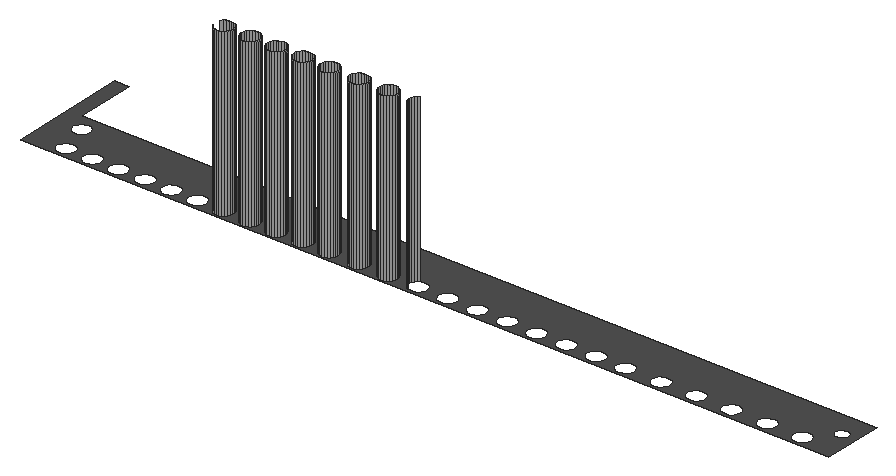
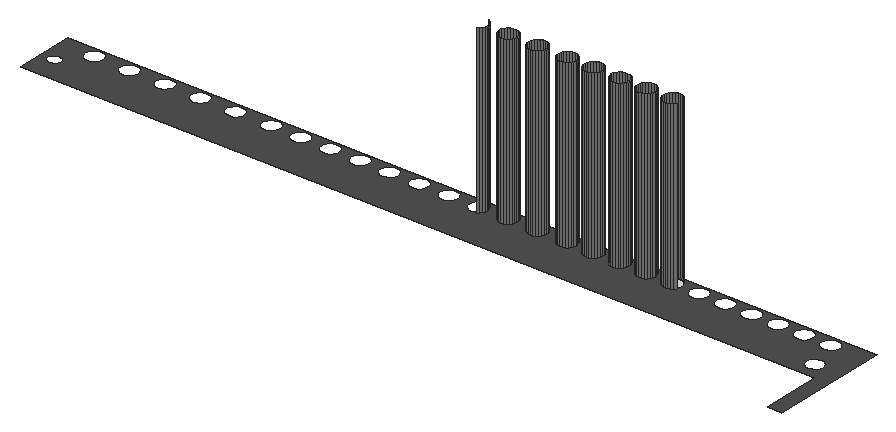
# SketchUp Ruby script. Lengths in inches.
U = 1.inch
M = Sketchup.active_model
def pt(a) = Geom::Point3d.new(a.map { |v| v * U })
def face(e, loops, mat)
  f = e.add_face(loops[0].map { |a| pt(a) })
  loops[1..].each { |l| e.add_face(l.map { |a| pt(a) }).erase! }
  f.material = f.back_material = mat if mat
  f
end
# faces: each face lists its corners as indices into pts; further lists are holes
def faces(e, pts, list, mat = nil) = list.each { |f| face(e, (f[0].is_a?(Array) ? f : [f]).map { |l| l.map { |i| pts[i] } }, mat) }
# xy, xz, yz: faces in a plane at the given z, y or x. An outline is a flat list of corners, or four numbers for a rectangle; further outlines are holes
def ring(l) = l.size == 4 ? [[l[0], l[1]], [l[2], l[1]], [l[2], l[3]], [l[0], l[3]]] : l.each_slice(2).to_a
def flat(e, list, mat, &to3) = list.each { |f| face(e, (f[0].is_a?(Array) ? f : [f]).map { |l| ring(l).map { |u, v| to3.(u, v) } }, mat) }
def xy(e, z, list, mat = nil) = flat(e, list, mat) { |x, y| [x, y, z] }
def xz(e, y, list, mat = nil) = flat(e, list, mat) { |x, z| [x, y, z] }
def yz(e, x, list, mat = nil) = flat(e, list, mat) { |y, z| [x, y, z] }
def lines(e, pts, list) = list.each { |a, b| e.add_line(pt(pts[a]), pt(pts[b])) }
# prism: a flat outline (further loops are holes) pulled along v
def prism(e, loops, v, mat = nil)
  f = face(e, loops, mat); d = Geom::Vector3d.new(v.map { |x| x * U })
  f.pushpull(f.normal.samedirection?(d) ? d.length : -d.length)
end
def box(e, o, s, mat = nil) = prism(e, [[o, [o[0] + s[0], o[1], o[2]], [o[0] + s[0], o[1] + s[1], o[2]], [o[0], o[1] + s[1], o[2]]]], [0, 0, s[2]], mat)
def at(x, y, z, deg = 0) = Geom::Transformation.translation(pt([x, y, z])) * Geom::Transformation.rotation(ORIGIN, Z_AXIS, deg.degrees)
def axes(o, x, y, z) = Geom::Transformation.new([*x, 0, *y, 0, *z, 0, *pt(o).to_a, 1])
def part(name) = M.definitions.add(name)
# library, detail: a bought-in or finely detailed component or shape, given as its bounding box
def library(name, o, s) = part(name).tap { |d| box(d.entities, o, s) }
def detail(e, o, s) = box(e.add_group.entities, o, s)
def put(e, d, t, mat = nil) = e.add_instance(d, t).tap { |i| i.material = mat if mat }
def group(e, t, mat = nil) = e.add_group.tap { |g| g.transformation = t; g.material = mat if mat }.entities
root = M.entities
M.materials.add("[0132_LightGray]").color = [169, 169, 169]
M.materials.add("[0135_DarkGray]").color = [81, 81, 81]
xy(root,638.72,[[270.33,31.93,269.97,31.97,269.64,32.11,269.36,32.33,269.14,32.62,269,32.95,268.95,33.3,269,33.66,269.14,33.99,269.36,34.28,269.64,34.49,269.97,34.63,270.33,34.68,270.68,34.63,271.02,34.49,271.3,34.28,271.52,33.99,271.66,33.66,271.7,33.3,271.66,32.95,271.52,32.62,271.3,32.33,271.02,32.11,270.68,31.97],[274.33,31.93,273.97,31.97,273.64,32.11,273.36,32.33,273.14,32.62,273,32.95,272.95,33.3,273,33.66,273.14,33.99,273.36,34.28,273.64,34.49,273.97,34.63,274.33,34.68,274.68,34.63,275.02,34.49,275.3,34.28,275.52,33.99,275.66,33.66,275.7,33.3,275.66,32.95,275.52,32.62,275.3,32.33,275.02,32.11,274.68,31.97],[278.33,31.93,277.97,31.97,277.64,32.11,277.36,32.33,277.14,32.62,277,32.95,276.95,33.3,277,33.66,277.14,33.99,277.36,34.28,277.64,34.49,277.97,34.63,278.33,34.68,278.68,34.63,279.02,34.49,279.3,34.28,279.52,33.99,279.66,33.66,279.7,33.3,279.66,32.95,279.52,32.62,279.3,32.33,279.02,32.11,278.68,31.97],[282.33,31.93,281.97,31.97,281.64,32.11,281.36,32.33,281.14,32.62,281,32.95,280.95,33.3,281,33.66,281.14,33.99,281.36,34.28,281.64,34.49,281.97,34.63,282.33,34.68,282.68,34.63,283.02,34.49,283.3,34.28,283.52,33.99,283.66,33.66,283.7,33.3,283.66,32.95,283.52,32.62,283.3,32.33,283.02,32.11,282.68,31.97],[286.33,31.93,285.97,31.97,285.64,32.11,285.36,32.33,285.14,32.62,285,32.95,284.95,33.3,285,33.66,285.14,33.99,285.36,34.28,285.64,34.49,285.97,34.63,286.33,34.68,286.68,34.63,287.02,34.49,287.3,34.28,287.52,33.99,287.66,33.66,287.7,33.3,287.66,32.95,287.52,32.62,287.3,32.33,287.02,32.11,286.68,31.97],
  [290.83,31.93,290.47,31.97,290.14,32.11,289.86,32.33,289.64,32.62,289.5,32.95,289.45,33.3,289.5,33.66,289.64,33.99,289.86,34.28,290.14,34.49,290.47,34.63,290.83,34.68,291.18,34.63,291.52,34.49,291.8,34.28,292.02,33.99,292.16,33.66,292.2,33.3,292.16,32.95,292.02,32.62,291.8,32.33,291.52,32.11,291.18,31.97],[295.33,31.93,294.97,31.97,294.64,32.11,294.36,32.33,294.14,32.62,294,32.95,293.95,33.3,294,33.66,294.14,33.99,294.36,34.28,294.64,34.49,294.97,34.63,295.33,34.68,295.68,34.63,296.02,34.49,296.3,34.28,296.52,33.99,296.66,33.66,296.7,33.3,296.66,32.95,296.52,32.62,296.3,32.33,296.02,32.11,295.68,31.97]])
xy(root,638.72,[[[240.7,31.6875,363.51,31.6875,363.51,40.6875,242.82,40.6875,242.82,49.6875,240.7,49.6875],[246.33,31.93,245.97,31.97,245.64,32.11,245.36,32.33,245.14,32.62,245,32.95,244.95,33.3,245,33.66,245.14,33.99,245.36,34.28,245.64,34.49,245.97,34.63,246.33,34.68,246.68,34.63,247.02,34.49,247.3,34.28,247.52,33.99,247.66,33.66,247.7,33.3,247.66,32.95,247.52,32.62,247.3,32.33,247.02,32.11,246.68,31.97],[250.33,31.93,249.97,31.97,249.64,32.11,249.36,32.33,249.14,32.62,249,32.95,248.95,33.3,249,33.66,249.14,33.99,249.36,34.28,249.64,34.49,249.97,34.63,250.33,34.68,250.68,34.63,251.02,34.49,251.3,34.28,251.52,33.99,251.66,33.66,251.7,33.3,251.66,32.95,251.52,32.62,251.3,32.33,251.02,32.11,250.68,31.97],[254.33,31.93,253.97,31.97,253.64,32.11,253.36,32.33,253.14,32.62,253,32.95,252.95,33.3,253,33.66,253.14,33.99,253.36,34.28,253.64,34.49,253.97,34.63,254.33,34.68,254.68,34.63,255.02,34.49,255.3,34.28,255.52,33.99,255.66,33.66,255.7,33.3,255.66,32.95,255.52,32.62,255.3,32.33,255.02,32.11,254.68,31.97],[258.33,31.93,257.97,31.97,257.64,32.11,257.36,32.33,257.14,32.62,257,32.95,256.95,33.3,257,33.66,257.14,33.99,257.36,34.28,257.64,34.49,257.97,34.63,258.33,34.68,258.68,34.63,259.02,34.49,259.3,34.28,259.52,33.99,259.66,33.66,259.7,33.3,259.66,32.95,259.52,32.62,259.3,32.33,259.02,32.11,258.68,31.97],[262.33,31.93,261.97,31.97,261.64,32.11,261.36,32.33,261.14,32.62,261,32.95,260.95,33.3,261,33.66,261.14,33.99,261.36,34.28,261.64,34.49,261.97,34.63,262.33,34.68,262.68,34.63,263.02,34.49,263.3,34.28,263.52,33.99,263.66,33.66,263.7,33.3,263.66,32.95,263.52,32.62,263.3,32.33,263.02,32.11,262.68,31.97],[266.33,31.93,265.97,31.97,265.64,32.11,265.36,32.33,265.14,32.62,265,32.95,264.95,33.3,265,33.66,265.14,33.99,265.36,34.28,265.64,34.49,265.97,34.63,266.33,34.68,266.68,34.63,267.02,34.49,267.3,34.28,267.52,33.99,267.66,33.66,267.7,33.3,267.66,32.95,267.52,32.62,267.3,32.33,267.02,32.11,266.68,31.97],[270.33,31.93,269.97,31.97,269.64,32.11,269.36,32.33,269.14,32.62,269,32.95,268.95,33.3,269,33.66,269.14,33.99,269.36,34.28,269.64,34.49,269.97,34.63,270.33,34.68,270.68,34.63,271.02,34.49,271.3,34.28,271.52,33.99,271.66,33.66,271.7,33.3,271.66,32.95,271.52,32.62,271.3,32.33,271.02,32.11,270.68,31.97],[274.33,31.93,273.97,31.97,273.64,32.11,273.36,32.33,273.14,32.62,273,32.95,272.95,33.3,273,33.66,273.14,33.99,273.36,34.28,273.64,34.49,273.97,34.63,274.33,34.68,274.68,34.63,275.02,34.49,275.3,34.28,275.52,33.99,275.66,33.66,275.7,33.3,275.66,32.95,275.52,32.62,275.3,32.33,275.02,32.11,274.68,31.97],[278.33,31.93,277.97,31.97,277.64,32.11,277.36,32.33,277.14,32.62,277,32.95,276.95,33.3,277,33.66,277.14,33.99,277.36,34.28,277.64,34.49,277.97,34.63,278.33,34.68,278.68,34.63,279.02,34.49,279.3,34.28,279.52,33.99,279.66,33.66,279.7,33.3,279.66,32.95,279.52,32.62,279.3,32.33,279.02,32.11,278.68,31.97],[282.33,31.93,281.97,31.97,281.64,32.11,281.36,32.33,281.14,32.62,281,32.95,280.95,33.3,281,33.66,281.14,33.99,281.36,34.28,281.64,34.49,281.97,34.63,282.33,34.68,282.68,34.63,283.02,34.49,283.3,34.28,283.52,33.99,283.66,33.66,283.7,33.3,283.66,32.95,283.52,32.62,283.3,32.33,283.02,32.11,282.68,31.97],[286.33,31.93,285.97,31.97,285.64,32.11,285.36,32.33,285.14,32.62,285,32.95,284.95,33.3,285,33.66,285.14,33.99,285.36,34.28,285.64,34.49,285.97,34.63,286.33,34.68,286.68,34.63,287.02,34.49,287.3,34.28,287.52,33.99,287.66,33.66,287.7,33.3,287.66,32.95,287.52,32.62,287.3,32.33,287.02,32.11,286.68,31.97],[290.83,31.93,290.47,31.97,290.14,32.11,289.86,32.33,289.64,32.62,289.5,32.95,289.45,33.3,289.5,33.66,289.64,33.99,289.86,34.28,290.14,34.49,290.47,34.63,290.83,34.68,291.18,34.63,291.52,34.49,291.8,34.28,292.02,33.99,292.16,33.66,292.2,33.3,292.16,32.95,292.02,32.62,291.8,32.33,291.52,32.11,291.18,31.97],[295.33,31.93,294.97,31.97,294.64,32.11,294.36,32.33,294.14,32.62,294,32.95,293.95,33.3,294,33.66,294.14,33.99,294.36,34.28,294.64,34.49,294.97,34.63,295.33,34.68,295.68,34.63,296.02,34.49,296.3,34.28,296.52,33.99,296.66,33.66,296.7,33.3,296.66,32.95,296.52,32.62,296.3,32.33,296.02,32.11,295.68,31.97],[299.83,31.93,299.47,31.97,299.14,32.11,298.86,32.33,298.64,32.62,298.5,32.95,298.45,33.3,298.5,33.66,298.64,33.99,298.86,34.28,299.14,34.49,299.47,34.63,299.83,34.68,300.18,34.63,300.52,34.49,300.8,34.28,301.02,33.99,301.16,33.66,301.2,33.3,301.16,32.95,301.02,32.62,300.8,32.33,300.52,32.11,300.18,31.97],[304.33,31.93,303.97,31.97,303.64,32.11,303.36,32.33,303.14,32.62,303,32.95,302.95,33.3,303,33.66,303.14,33.99,303.36,34.28,303.64,34.49,303.97,34.63,304.33,34.68,304.68,34.63,305.02,34.49,305.3,34.28,305.52,33.99,305.66,33.66,305.7,33.3,305.66,32.95,305.52,32.62,305.3,32.33,305.02,32.11,304.68,31.97],[308.83,31.93,308.47,31.97,308.14,32.11,307.86,32.33,307.64,32.62,307.5,32.95,307.45,33.3,307.5,33.66,307.64,33.99,307.86,34.28,308.14,34.49,308.47,34.63,308.83,34.68,309.18,34.63,309.52,34.49,309.8,34.28,310.02,33.99,310.16,33.66,310.2,33.3,310.16,32.95,310.02,32.62,309.8,32.33,309.52,32.11,309.18,31.97],[313.33,31.93,312.97,31.97,312.64,32.11,312.36,32.33,312.14,32.62,312,32.95,311.95,33.3,312,33.66,312.14,33.99,312.36,34.28,312.64,34.49,312.97,34.63,313.33,34.68,313.68,34.63,314.02,34.49,314.3,34.28,314.52,33.99,314.66,33.66,314.7,33.3,314.66,32.95,314.52,32.62,314.3,32.33,314.02,32.11,313.68,31.97],[317.83,31.93,317.47,31.97,317.14,32.11,316.86,32.33,316.64,32.62,316.5,32.95,316.45,33.3,316.5,33.66,316.64,33.99,316.86,34.28,317.14,34.49,317.47,34.63,317.83,34.68,318.18,34.63,318.52,34.49,318.8,34.28,319.02,33.99,319.16,33.66,319.2,33.3,319.16,32.95,319.02,32.62,318.8,32.33,318.52,32.11,318.18,31.97],[322.33,31.93,321.97,31.97,321.64,32.11,321.36,32.33,321.14,32.62,321,32.95,320.95,33.3,321,33.66,321.14,33.99,321.36,34.28,321.64,34.49,321.97,34.63,322.33,34.68,322.68,34.63,323.02,34.49,323.3,34.28,323.52,33.99,323.66,33.66,323.7,33.3,323.66,32.95,323.52,32.62,323.3,32.33,323.02,32.11,322.68,31.97],[326.83,31.93,326.47,31.97,326.14,32.11,325.86,32.33,325.64,32.62,325.5,32.95,325.45,33.3,325.5,33.66,325.64,33.99,325.86,34.28,326.14,34.49,326.47,34.63,326.83,34.68,327.18,34.63,327.52,34.49,327.8,34.28,328.02,33.99,328.16,33.66,328.2,33.3,328.16,32.95,328.02,32.62,327.8,32.33,327.52,32.11,327.18,31.97],[331.33,31.93,330.97,31.97,330.64,32.11,330.36,32.33,330.14,32.62,330,32.95,329.95,33.3,330,33.66,330.14,33.99,330.36,34.28,330.64,34.49,330.97,34.63,331.33,34.68,331.68,34.63,332.02,34.49,332.3,34.28,332.52,33.99,332.66,33.66,332.7,33.3,332.66,32.95,332.52,32.62,332.3,32.33,332.02,32.11,331.68,31.97],[336.7,31.93,336.35,31.97,336.02,32.11,335.73,32.33,335.51,32.62,335.375,32.95,335.33,33.3,335.375,33.66,335.51,33.99,335.73,34.28,336.02,34.49,336.35,34.63,336.7,34.68,337.06,34.63,337.39,34.49,337.68,34.28,337.89,33.99,338.03,33.66,338.08,33.3,338.03,32.95,337.89,32.62,337.68,32.33,337.39,32.11,337.06,31.97],[342.08,31.93,341.72,31.97,341.39,32.11,341.11,32.33,340.89,32.62,340.75,32.95,340.7,33.3,340.75,33.66,340.89,33.99,341.11,34.28,341.39,34.49,341.72,34.63,342.08,34.68,342.43,34.63,342.77,34.49,343.05,34.28,343.27,33.99,343.41,33.66,343.45,33.3,343.41,32.95,343.27,32.62,343.05,32.33,342.77,32.11,342.43,31.97],[347.45,31.93,347.1,31.97,346.77,32.11,346.48,32.33,346.26,32.62,346.125,32.95,346.08,33.3,346.125,33.66,346.26,33.99,346.48,34.28,346.77,34.49,347.1,34.63,347.45,34.68,347.81,34.63,348.14,34.49,348.43,34.28,348.64,33.99,348.78,33.66,348.83,33.3,348.78,32.95,348.64,32.62,348.43,32.33,348.14,32.11,347.81,31.97],[352.83,31.93,352.47,31.97,352.14,32.11,351.86,32.33,351.64,32.62,351.5,32.95,351.45,33.3,351.5,33.66,351.64,33.99,351.86,34.28,352.14,34.49,352.47,34.63,352.83,34.68,353.18,34.63,353.52,34.49,353.8,34.28,354.02,33.99,354.16,33.66,354.2,33.3,354.16,32.95,354.02,32.62,353.8,32.33,353.52,32.11,353.18,31.97],[358.2,31.93,357.85,31.97,357.52,32.11,357.23,32.33,357.01,32.62,356.875,32.95,356.83,33.3,356.875,33.66,357.01,33.99,357.23,34.28,357.52,34.49,357.85,34.63,358.2,34.68,358.56,34.63,358.89,34.49,359.18,34.28,359.39,33.99,359.53,33.66,359.58,33.3,359.53,32.95,359.39,32.62,359.18,32.33,358.89,32.11,358.56,31.97],[244.88,36.8,244.54,36.84,244.22,36.97,243.95,37.18,243.74,37.45,243.61,37.77,243.57,38.11,243.61,38.45,243.74,38.77,243.95,39.04,244.22,39.25,244.54,39.38,244.88,39.42,245.22,39.38,245.53,39.25,245.81,39.04,246.01,38.77,246.15,38.45,246.19,38.11,246.15,37.77,246.01,37.45,245.81,37.18,245.53,36.97,245.22,36.84],[361.31,35.875,361.05,35.93,360.82,36.05,360.62,36.22,360.48,36.4375,360.4,36.6875,360.38,36.95,360.4375,37.2,360.55,37.4375,360.73,37.63,360.95,37.77,361.19,37.85,361.46,37.87,361.71,37.82,361.94,37.7,362.14,37.52,362.28,37.31,362.36,37.06,362.38,36.8,362.32,36.54,362.21,36.31,362.03,36.11,361.8125,35.97,361.57,35.89]]],"[0135_DarkGray]")
p = [[269.97,31.97,638.72],[270.33,31.93,638.72],[270.33,31.93,663.85],[269.97,31.97,663.85],[270.68,31.97,638.72],[270.68,31.97,663.85],
  [273.97,31.97,638.72],[274.33,31.93,638.72],[274.33,31.93,663.85],[273.97,31.97,663.85],[274.68,31.97,638.72],[274.68,31.97,663.85],
  [277.97,31.97,638.72],[278.33,31.93,638.72],[278.33,31.93,663.85],[277.97,31.97,663.85],[278.68,31.97,638.72],[278.68,31.97,663.85],
  [281.97,31.97,638.72],[282.33,31.93,638.72],[282.33,31.93,663.85],[281.97,31.97,663.85],[282.68,31.97,638.72],[282.68,31.97,663.85],
  [285.97,31.97,638.72],[286.33,31.93,638.72],[286.33,31.93,663.85],[285.97,31.97,663.85],[286.68,31.97,638.72],[286.68,31.97,663.85],
  [290.47,31.97,638.72],[290.83,31.93,638.72],[290.83,31.93,663.85],[290.47,31.97,663.85],[291.18,31.97,638.72],[291.18,31.97,663.85],
  [294.97,31.97,638.72],[295.33,31.93,638.72],[295.33,31.93,663.85],[294.97,31.97,663.85],[295.68,31.97,638.72],[295.68,31.97,663.85],
  [269.64,32.11,638.72],[269.64,32.11,663.85],[271.02,32.11,638.72],[271.02,32.11,663.85],[273.64,32.11,638.72],[273.64,32.11,663.85],
  [275.02,32.11,638.72],[275.02,32.11,663.85],[277.64,32.11,638.72],[277.64,32.11,663.85],[279.02,32.11,638.72],[279.02,32.11,663.85],
  [281.64,32.11,638.72],[281.64,32.11,663.85],[283.02,32.11,638.72],[283.02,32.11,663.85],[285.64,32.11,638.72],[285.64,32.11,663.85],
  [287.02,32.11,638.72],[287.02,32.11,663.85],[290.14,32.11,638.72],[290.14,32.11,663.85],[291.52,32.11,638.72],[291.52,32.11,663.85],
  [294.64,32.11,638.72],[294.64,32.11,663.85],[296.02,32.11,638.72],[296.02,32.11,663.85],[269.36,32.33,638.72],[269.36,32.33,663.85],
  [271.3,32.33,638.72],[271.3,32.33,663.85],[273.36,32.33,638.72],[273.36,32.33,663.85],[275.3,32.33,638.72],[275.3,32.33,663.85],
  [277.36,32.33,638.72],[277.36,32.33,663.85],[279.3,32.33,638.72],[279.3,32.33,663.85],[281.36,32.33,638.72],[281.36,32.33,663.85],
  [283.3,32.33,638.72],[283.3,32.33,663.85],[285.36,32.33,638.72],[285.36,32.33,663.85],[287.3,32.33,638.72],[287.3,32.33,663.85],
  [289.86,32.33,638.72],[289.86,32.33,663.85],[291.8,32.33,638.72],[291.8,32.33,663.85],[294.36,32.33,638.72],[294.36,32.33,663.85],
  [296.3,32.33,638.72],[296.3,32.33,663.85],[298.86,32.33,638.72],[299.14,32.11,638.72],[299.14,32.11,663.85],[298.86,32.33,663.85],
  [269.14,32.62,638.72],[269.14,32.62,663.85],[271.52,32.62,638.72],[271.52,32.62,663.85],[273.14,32.62,638.72],[273.14,32.62,663.85],
  [275.52,32.62,638.72],[275.52,32.62,663.85],[277.14,32.62,638.72],[277.14,32.62,663.85],[279.52,32.62,638.72],[279.52,32.62,663.85],
  [281.14,32.62,638.72],[281.14,32.62,663.85],[283.52,32.62,638.72],[283.52,32.62,663.85],[285.14,32.62,638.72],[285.14,32.62,663.85],
  [287.52,32.62,638.72],[287.52,32.62,663.85],[289.64,32.62,638.72],[289.64,32.62,663.85],[292.02,32.62,638.72],[292.02,32.62,663.85],
  [294.14,32.62,638.72],[294.14,32.62,663.85],[296.52,32.62,638.72],[296.52,32.62,663.85],[298.64,32.62,638.72],[298.64,32.62,663.85],
  [271.66,32.95,638.72],[271.66,32.95,663.85],[273,32.95,638.72],[273,32.95,663.85],[275.66,32.95,638.72],[275.66,32.95,663.85],
  [277,32.95,638.72],[277,32.95,663.85],[279.66,32.95,638.72],[279.66,32.95,663.85],[281,32.95,638.72],[281,32.95,663.85],
  [283.66,32.95,638.72],[283.66,32.95,663.85],[285,32.95,638.72],[285,32.95,663.85],[287.66,32.95,638.72],[287.66,32.95,663.85],
  [289.5,32.95,638.72],[289.5,32.95,663.85],[292.16,32.95,638.72],[292.16,32.95,663.85],[294,32.95,638.72],[294,32.95,663.85],
  [296.66,32.95,638.72],[296.66,32.95,663.85],[298.5,32.95,638.72],[298.5,32.95,663.85],[271.7,33.3,638.72],[271.7,33.3,663.85],
  [272.95,33.3,638.72],[272.95,33.3,663.85],[275.7,33.3,638.72],[275.7,33.3,663.85],[276.95,33.3,638.72],[276.95,33.3,663.85],
  [279.7,33.3,638.72],[279.7,33.3,663.85],[280.95,33.3,638.72],[280.95,33.3,663.85],[283.7,33.3,638.72],[283.7,33.3,663.85],
  [284.95,33.3,638.72],[284.95,33.3,663.85],[287.7,33.3,638.72],[287.7,33.3,663.85],[289.45,33.3,638.72],[289.45,33.3,663.85],
  [292.2,33.3,638.72],[292.2,33.3,663.85],[293.95,33.3,638.72],[293.95,33.3,663.85],[296.7,33.3,638.72],[296.7,33.3,663.85],
  [298.45,33.3,638.72],[298.45,33.3,663.85],[271.66,33.66,638.72],[271.66,33.66,663.85],[273,33.66,638.72],[273,33.66,663.85],
  [275.66,33.66,638.72],[275.66,33.66,663.85],[277,33.66,638.72],[277,33.66,663.85],[279.66,33.66,638.72],[279.66,33.66,663.85],
  [281,33.66,638.72],[281,33.66,663.85],[283.66,33.66,638.72],[283.66,33.66,663.85],[285,33.66,638.72],[285,33.66,663.85],
  [287.66,33.66,638.72],[287.66,33.66,663.85],[289.5,33.66,638.72],[289.5,33.66,663.85],[292.16,33.66,638.72],[292.16,33.66,663.85],
  [294,33.66,638.72],[294,33.66,663.85],[296.66,33.66,638.72],[296.66,33.66,663.85],[298.5,33.66,638.72],[298.5,33.66,663.85],
  [271.52,33.99,638.72],[271.52,33.99,663.85],[273.14,33.99,638.72],[273.14,33.99,663.85],[275.52,33.99,638.72],[275.52,33.99,663.85],
  [277.14,33.99,638.72],[277.14,33.99,663.85],[279.52,33.99,638.72],[279.52,33.99,663.85],[281.14,33.99,638.72],[281.14,33.99,663.85],
  [283.52,33.99,638.72],[283.52,33.99,663.85],[285.14,33.99,638.72],[285.14,33.99,663.85],[287.52,33.99,638.72],[287.52,33.99,663.85],
  [289.64,33.99,638.72],[289.64,33.99,663.85],[292.02,33.99,638.72],[292.02,33.99,663.85],[294.14,33.99,638.72],[294.14,33.99,663.85],
  [296.52,33.99,638.72],[296.52,33.99,663.85],[298.64,33.99,638.72],[298.64,33.99,663.85],[269.36,34.28,638.72],[269.14,33.99,638.72],
  [269.14,33.99,663.85],[269.36,34.28,663.85],[271.3,34.28,638.72],[271.3,34.28,663.85],[273.36,34.28,638.72],[273.36,34.28,663.85],
  [275.3,34.28,638.72],[275.3,34.28,663.85],[277.36,34.28,638.72],[277.36,34.28,663.85],[279.3,34.28,638.72],[279.3,34.28,663.85],
  [281.36,34.28,638.72],[281.36,34.28,663.85],[283.3,34.28,638.72],[283.3,34.28,663.85],[285.36,34.28,638.72],[285.36,34.28,663.85],
  [287.3,34.28,638.72],[287.3,34.28,663.85],[289.86,34.28,638.72],[289.86,34.28,663.85],[291.8,34.28,638.72],[291.8,34.28,663.85],
  [294.36,34.28,638.72],[294.36,34.28,663.85],[296.3,34.28,638.72],[296.3,34.28,663.85],[298.86,34.28,638.72],[298.86,34.28,663.85],
  [269.64,34.49,638.72],[269.64,34.49,663.85],[271.02,34.49,638.72],[271.02,34.49,663.85],[273.64,34.49,638.72],[273.64,34.49,663.85],
  [275.02,34.49,638.72],[275.02,34.49,663.85],[277.64,34.49,638.72],[277.64,34.49,663.85],[279.02,34.49,638.72],[279.02,34.49,663.85],
  [281.64,34.49,638.72],[281.64,34.49,663.85],[283.02,34.49,638.72],[283.02,34.49,663.85],[285.64,34.49,638.72],[285.64,34.49,663.85],
  [287.02,34.49,638.72],[287.02,34.49,663.85],[290.14,34.49,638.72],[290.14,34.49,663.85],[291.52,34.49,638.72],[291.52,34.49,663.85],
  [294.64,34.49,638.72],[294.64,34.49,663.85],[296.02,34.49,638.72],[296.02,34.49,663.85],[299.14,34.49,638.72],[299.14,34.49,663.85],
  [269.97,34.63,638.72],[269.97,34.63,663.85],[270.68,34.63,638.72],[270.68,34.63,663.85],[273.97,34.63,638.72],[273.97,34.63,663.85],
  [274.68,34.63,638.72],[274.68,34.63,663.85],[277.97,34.63,638.72],[277.97,34.63,663.85],[278.68,34.63,638.72],[278.68,34.63,663.85],
  [281.97,34.63,638.72],[281.97,34.63,663.85],[282.68,34.63,638.72],[282.68,34.63,663.85],[285.97,34.63,638.72],[285.97,34.63,663.85],
  [286.68,34.63,638.72],[286.68,34.63,663.85],[290.47,34.63,638.72],[290.47,34.63,663.85],[291.18,34.63,638.72],[291.18,34.63,663.85],
  [294.97,34.63,638.72],[294.97,34.63,663.85],[295.68,34.63,638.72],[295.68,34.63,663.85],[270.33,34.68,638.72],[270.33,34.68,663.85],
  [274.33,34.68,638.72],[274.33,34.68,663.85],[278.33,34.68,638.72],[278.33,34.68,663.85],[282.33,34.68,638.72],[282.33,34.68,663.85],
  [286.33,34.68,638.72],[286.33,34.68,663.85],[290.83,34.68,638.72],[290.83,34.68,663.85],[295.33,34.68,638.72],[295.33,34.68,663.85]]
faces(root,p,[[0,1,2,3],[1,4,5,2],[6,7,8,9],[7,10,11,8],[12,13,14,15],[13,16,17,14],[18,19,20,21],[19,22,23,20],
  [24,25,26,27],[25,28,29,26],[30,31,32,33],[31,34,35,32],[36,37,38,39],[37,40,41,38],[42,0,3,43],[4,44,45,5],
  [46,6,9,47],[10,48,49,11],[50,12,15,51],[16,52,53,17],[54,18,21,55],[22,56,57,23],[58,24,27,59],[28,60,61,29],
  [62,30,33,63],[34,64,65,35],[66,36,39,67],[40,68,69,41],[70,42,43,71],[44,72,73,45],[74,46,47,75],[48,76,77,49],
  [78,50,51,79],[52,80,81,53],[82,54,55,83],[56,84,85,57],[86,58,59,87],[60,88,89,61],[90,62,63,91],[64,92,93,65],
  [94,66,67,95],[68,96,97,69],[98,99,100,101],[102,70,71,103],[72,104,105,73],[106,74,75,107],[76,108,109,77],[110,78,79,111],
  [80,112,113,81],[114,82,83,115],[84,116,117,85],[118,86,87,119],[88,120,121,89],[122,90,91,123],[92,124,125,93],[126,94,95,127],
  [96,128,129,97],[130,98,101,131],[104,132,133,105],[134,106,107,135],[108,136,137,109],[138,110,111,139],[112,140,141,113],[142,114,115,143],
  [116,144,145,117],[146,118,119,147],[120,148,149,121],[150,122,123,151],[124,152,153,125],[154,126,127,155],[128,156,157,129],[158,130,131,159],
  [132,160,161,133],[162,134,135,163],[136,164,165,137],[166,138,139,167],[140,168,169,141],[170,142,143,171],[144,172,173,145],[174,146,147,175],
  [148,176,177,149],[178,150,151,179],[152,180,181,153],[182,154,155,183],[156,184,185,157],[186,158,159,187],[160,188,189,161],[190,162,163,191],
  [164,192,193,165],[194,166,167,195],[168,196,197,169],[198,170,171,199],[172,200,201,173],[202,174,175,203],[176,204,205,177],[206,178,179,207],
  [180,208,209,181],[210,182,183,211],[184,212,213,185],[214,186,187,215],[188,216,217,189],[218,190,191,219],[192,220,221,193],[222,194,195,223],
  [196,224,225,197],[226,198,199,227],[200,228,229,201],[230,202,203,231],[204,232,233,205],[234,206,207,235],[208,236,237,209],[238,210,211,239],
  [212,240,241,213],[242,214,215,243],[244,245,246,247],[216,248,249,217],[250,218,219,251],[220,252,253,221],[254,222,223,255],[224,256,257,225],
  [258,226,227,259],[228,260,261,229],[262,230,231,263],[232,264,265,233],[266,234,235,267],[236,268,269,237],[270,238,239,271],[240,272,273,241],
  [274,242,243,275],[276,244,247,277],[248,278,279,249],[280,250,251,281],[252,282,283,253],[284,254,255,285],[256,286,287,257],[288,258,259,289],
  [260,290,291,261],[292,262,263,293],[264,294,295,265],[296,266,267,297],[268,298,299,269],[300,270,271,301],[272,302,303,273],[304,274,275,305],
  [306,276,277,307],[278,308,309,279],[310,280,281,311],[282,312,313,283],[314,284,285,315],[286,316,317,287],[318,288,289,319],[290,320,321,291],
  [322,292,293,323],[294,324,325,295],[326,296,297,327],[298,328,329,299],[330,300,301,331],[302,332,333,303],[334,306,307,335],[308,334,335,309],
  [336,310,311,337],[312,336,337,313],[338,314,315,339],[316,338,339,317],[340,318,319,341],[320,340,341,321],[342,322,323,343],[324,342,343,325],
  [344,326,327,345],[328,344,345,329],[346,330,331,347],[332,346,347,333]],"[0132_LightGray]")
